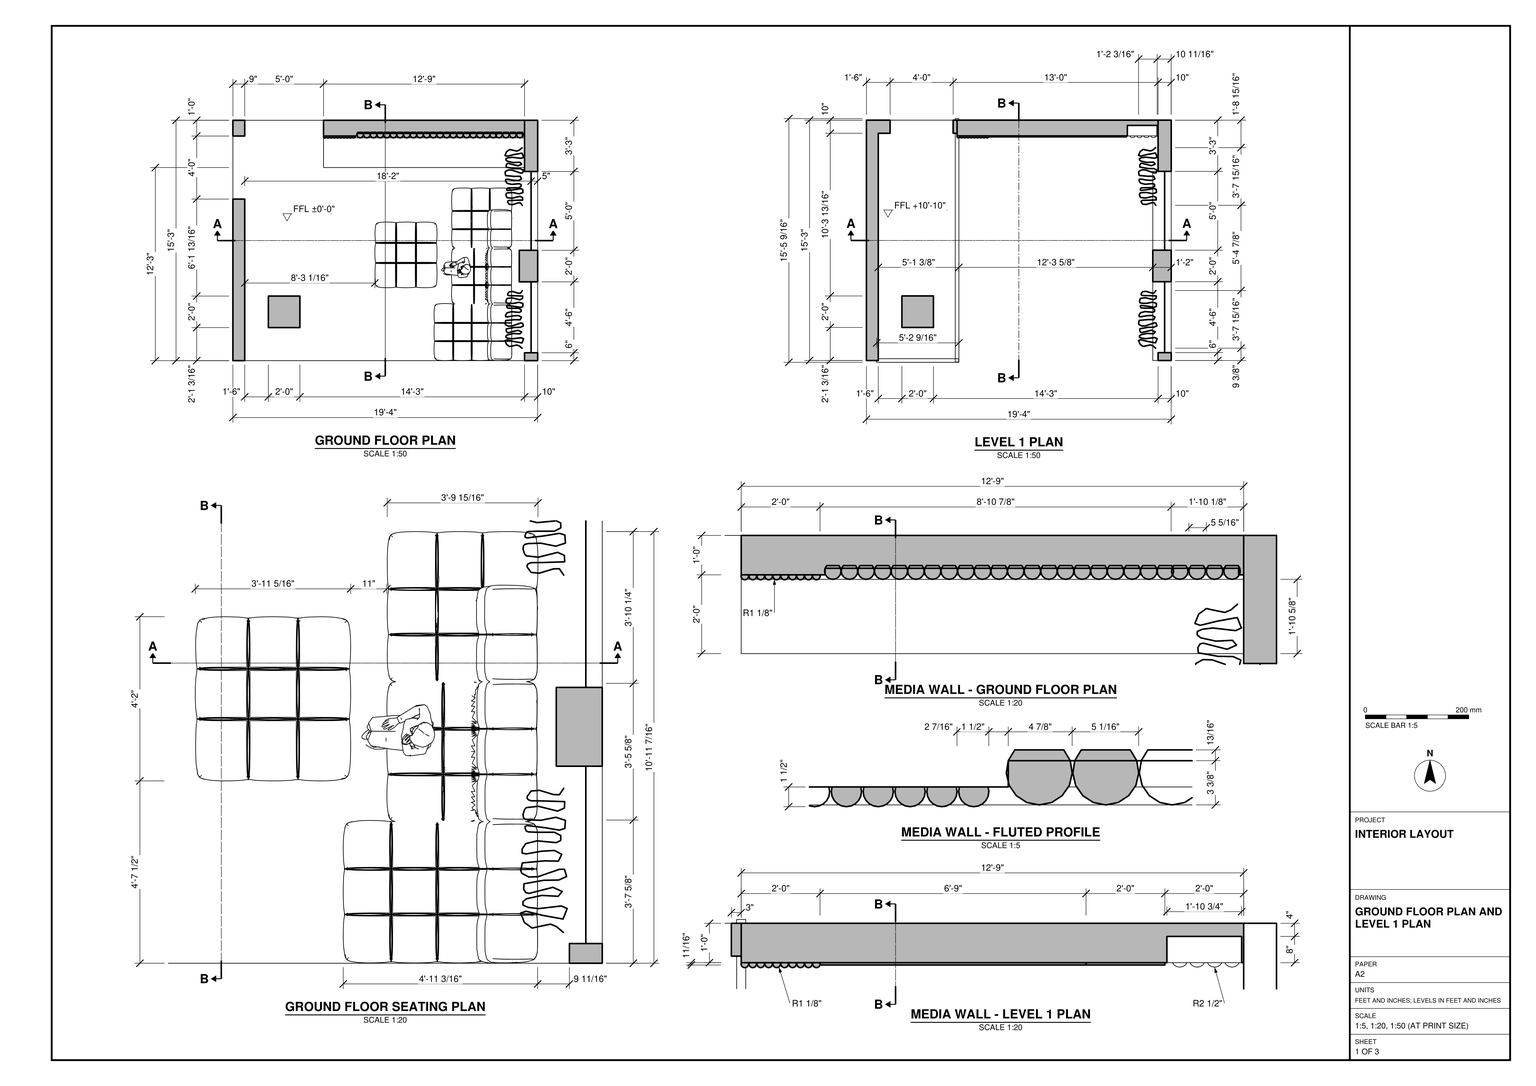
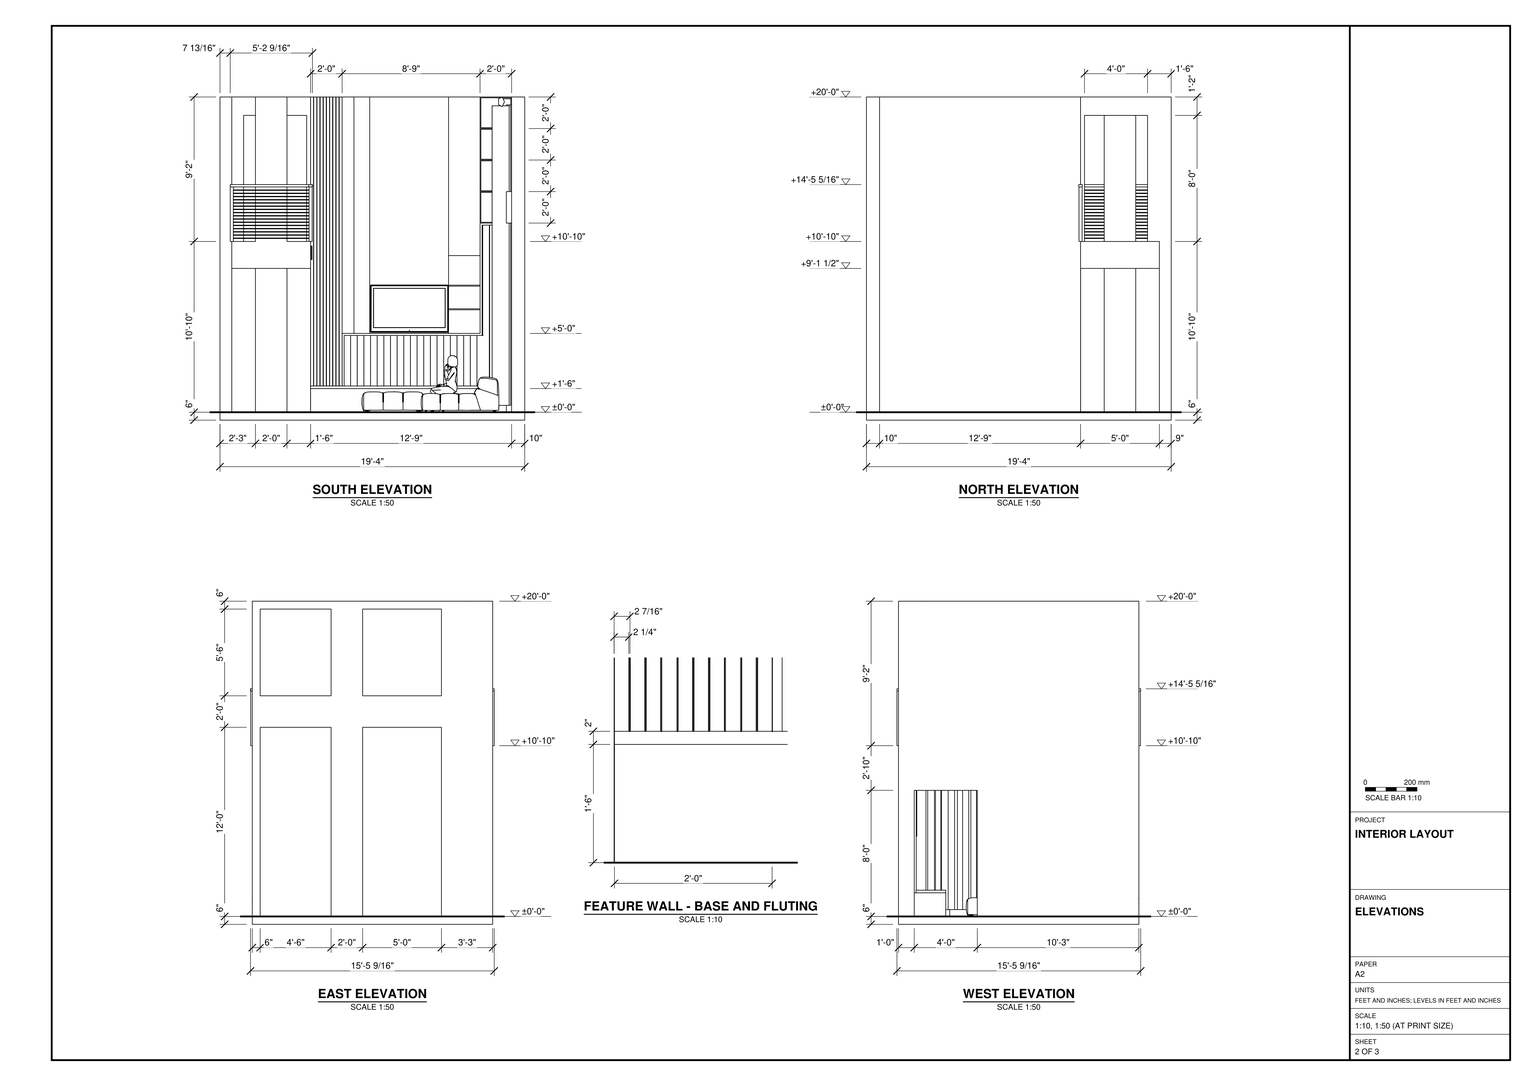
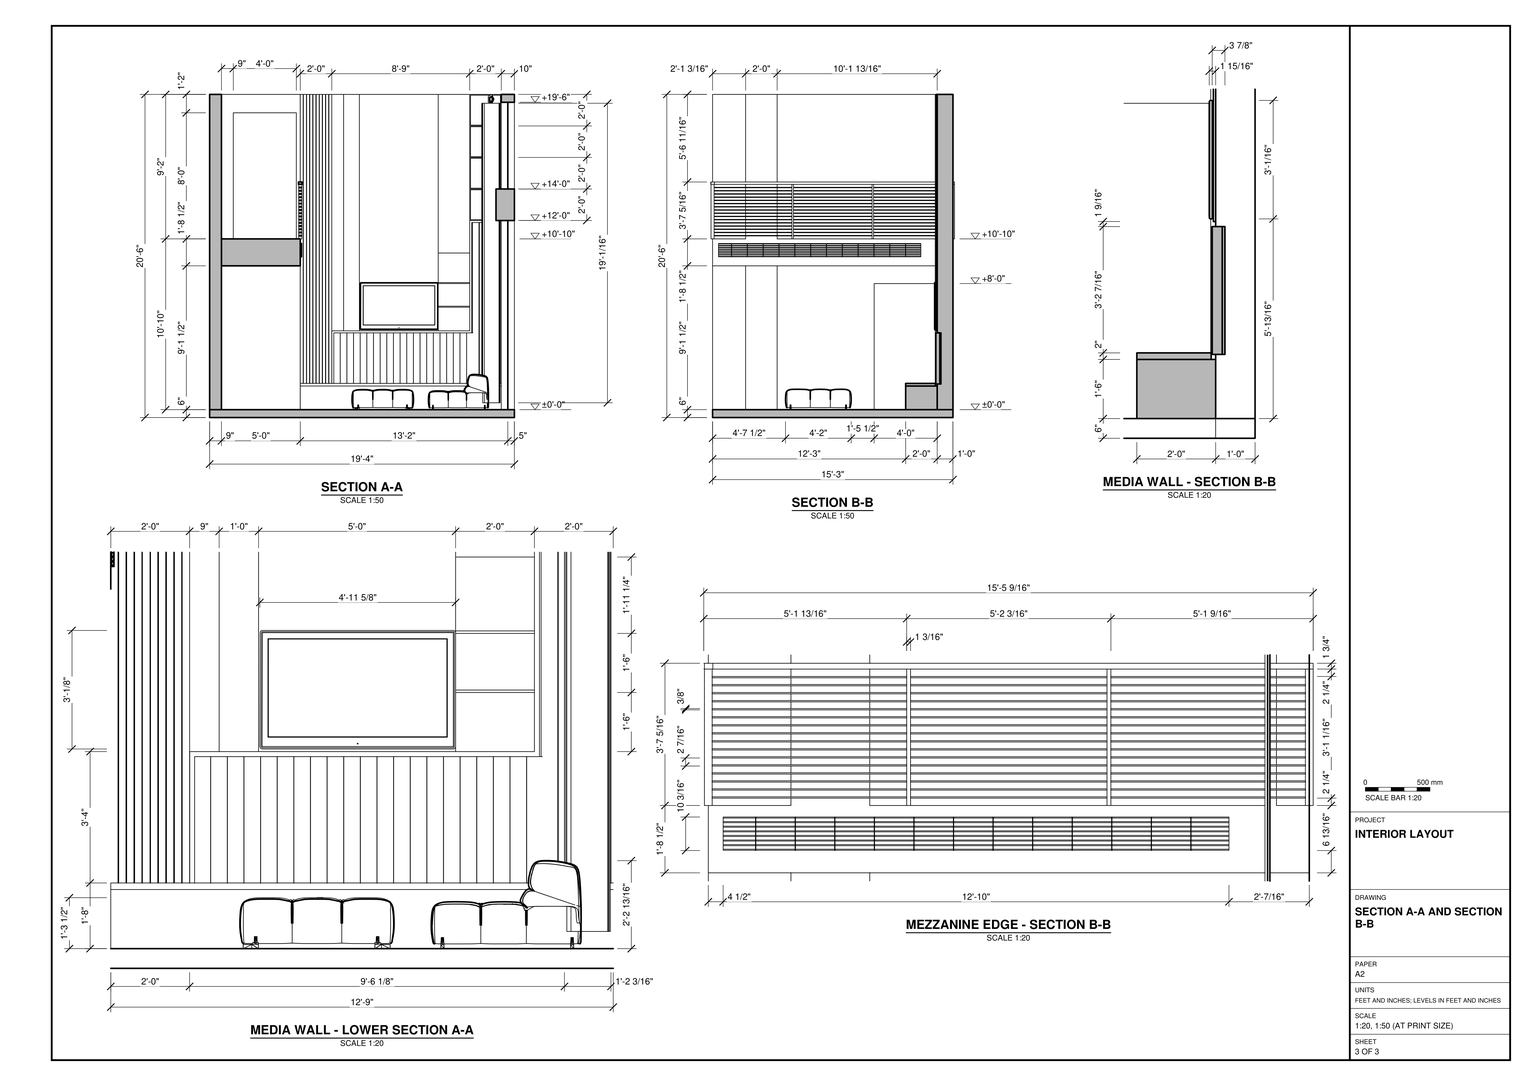
Build the lounge in SketchUp from task_files/diagram_01.pdf. Work in feet and inches. The overall model is 19'-4" wide, 15'-5 9/16" deep and 20'-6" high. Set the ground finished floor at ±0'-0" and the mezzanine finished floor at +10'-10". The overall height includes the 6" ground slab below the finished floor.

Use the plans to locate the walls, their returns and the square column. Match the wall thicknesses and opening sizes to the plans and elevations. Form the narrow mezzanine along the west side, leaving the seating area open to the full room height. Use the mezzanine edge detail to model the horizontal guard rails, their posts and the long grille in the fascia below them.

Build the north media wall in relief. Include the projecting plinth, the narrow full-height fluted strip, the broader flutes below the screen, the tall panels and the shelving beside the screen. Place the long sectional sofa along the east side, with its deeper end as drawn. Leave a gap between the sofa and the separate upholstered ottoman. Decor and loose items, including the curtains and screen, may be any suitable library components.

Keep shell elements and individual furniture or joinery pieces in separate groups or components, and use components for repeated parts. Save one SketchUp model as output_files/double_height_lounge_with_a_mezzanine_and_media_wall.skp.

# SketchUp Ruby script. Lengths in inches.
U = 1.inch
M = Sketchup.active_model
def pt(a) = Geom::Point3d.new(a.map { |v| v * U })
def face(e, loops, mat)
  f = e.add_face(loops[0].map { |a| pt(a) })
  loops[1..].each { |l| e.add_face(l.map { |a| pt(a) }).erase! }
  f.material = f.back_material = mat if mat
  f
end
# faces: each face lists its corners as indices into pts; further lists are holes
def faces(e, pts, list, mat = nil) = list.each { |f| face(e, (f[0].is_a?(Array) ? f : [f]).map { |l| l.map { |i| pts[i] } }, mat) }
# xy, xz, yz: faces in a plane at the given z, y or x. An outline is a flat list of corners, or four numbers for a rectangle; further outlines are holes
def ring(l) = l.size == 4 ? [[l[0], l[1]], [l[2], l[1]], [l[2], l[3]], [l[0], l[3]]] : l.each_slice(2).to_a
def flat(e, list, mat, &to3) = list.each { |f| face(e, (f[0].is_a?(Array) ? f : [f]).map { |l| ring(l).map { |u, v| to3.(u, v) } }, mat) }
def xy(e, z, list, mat = nil) = flat(e, list, mat) { |x, y| [x, y, z] }
def xz(e, y, list, mat = nil) = flat(e, list, mat) { |x, z| [x, y, z] }
def yz(e, x, list, mat = nil) = flat(e, list, mat) { |y, z| [x, y, z] }
def lines(e, pts, list) = list.each { |a, b| e.add_line(pt(pts[a]), pt(pts[b])) }
# prism: a flat outline (further loops are holes) pulled along v
def prism(e, loops, v, mat = nil)
  f = face(e, loops, mat); d = Geom::Vector3d.new(v.map { |x| x * U })
  f.pushpull(f.normal.samedirection?(d) ? d.length : -d.length)
end
def box(e, o, s, mat = nil) = prism(e, [[o, [o[0] + s[0], o[1], o[2]], [o[0] + s[0], o[1] + s[1], o[2]], [o[0], o[1] + s[1], o[2]]]], [0, 0, s[2]], mat)
def at(x, y, z, deg = 0) = Geom::Transformation.translation(pt([x, y, z])) * Geom::Transformation.rotation(ORIGIN, Z_AXIS, deg.degrees)
def axes(o, x, y, z) = Geom::Transformation.new([*x, 0, *y, 0, *z, 0, *pt(o).to_a, 1])
def part(name) = M.definitions.add(name)
# library, detail: a bought-in or finely detailed component or shape, given as its bounding box
def library(name, o, s) = part(name).tap { |d| box(d.entities, o, s) }
def detail(e, o, s) = box(e.add_group.entities, o, s)
def put(e, d, t, mat = nil) = e.add_instance(d, t).tap { |i| i.material = mat if mat }
def group(e, t, mat = nil) = e.add_group.tap { |g| g.transformation = t; g.material = mat if mat }.entities
root = M.entities
M.materials.add("1111 AP 9939 Brown seed-N").color = [122, 81, 68]
M.materials.add("FABRIC ARCHITEX BELLA OLD GOLD").color = [163, 137, 58]
M.materials.add("[Carrera Marble]").color = [206, 206, 206]
M.materials.add("[Color M06]").color = [86, 86, 86]
M.materials.add("[Color M08]").color = [30, 30, 30]
M.materials.add("[Color_D17]").color = [102, 81, 20]
M.materials.add("[Translucent Glass Gray]").color = [128, 128, 128]
M.materials["[Translucent Glass Gray]"].alpha = 0.5
M.materials.add("[Wood Cherry Original]").color = [152, 86, 42]
M.materials.add("[sketch-stone]").color = [126, 99, 107]
c1 = library("Sem nome",[3.92,4.36,0],[38.43,1.9,23.875])
c2 = part("d1")
xy(c2.entities,0,[[0,0,18,1.6],[18,0,36,1.6]],"[sketch-stone]")
xy(c2.entities,72,[[0,0,18,1.6],[18,0,36,1.6]],"[sketch-stone]")
yz(c2.entities,0,[[0,0,1.6,72]],"[sketch-stone]")
yz(c2.entities,36,[[0,0,1.6,72]],"[sketch-stone]")
c3 = part("元件\#28")
box(c3.entities,[0,0.12,0],[0.79,61.77,0.12])
c4 = part("元件\#29")
box(c4.entities,[0,0,0],[0.79,0.2,3.9375])
c5 = part("建立群組\#147")
box(c5.entities,[-0.38,0,0],[0.58,61.77,3.46],"[Color M06]")
c6 = part("建立群組\#1")
put(c6.entities,c3,axes([0,-0.29,0.66],[1.22759,0,0],[0,2.44422,0],[0,0,1.22686]))
put(c6.entities,c3,axes([0,-0.29,0.04],[1.22759,0,0],[0,2.44422,0],[0,0,1.22686]))
put(c6.entities,c4,axes([0.2,139.5625,0],[1.16,0,0],[0,0.66284,0],[0,0,1.16]))
put(c6.entities,c3,axes([0,-0.29,3.8],[1.22759,0,0],[0,2.44422,0],[0,0,1.22686]))
put(c6.entities,c3,axes([0,-0.29,2.55],[1.22759,0,0],[0,2.44422,0],[0,0,1.22686]))
put(c6.entities,c3,axes([0,-0.29,3.18],[1.22759,0,0],[0,2.44422,0],[0,0,1.22686]))
put(c6.entities,c3,axes([0,-0.29,1.29],[1.22759,0,0],[0,2.44422,0],[0,0,1.22686]))
put(c6.entities,c3,axes([0,-0.29,4.43],[1.22759,0,0],[0,2.44422,0],[0,0,1.22686]))
put(c6.entities,c3,axes([0,-0.29,1.92],[1.22759,0,0],[0,2.44422,0],[0,0,1.22686]))
put(c6.entities,c4,axes([0.2,80.51,0],[1.16,0,0],[0,0.66284,0],[0,0,1.16]))
put(c6.entities,c4,axes([0.2,56.88,0],[1.16,0,0],[0,0.66284,0],[0,0,1.16]))
put(c6.entities,c4,axes([0.2,45.07,0],[1.16,0,0],[0,0.66284,0],[0,0,1.16]))
put(c6.entities,c4,axes([0.2,21.45,0],[1.16,0,0],[0,0.66284,0],[0,0,1.16]))
put(c6.entities,c4,axes([0.2,127.75,0],[1.16,0,0],[0,0.66284,0],[0,0,1.16]))
put(c6.entities,c4,axes([0.2,115.9375,0],[1.16,0,0],[0,0.66284,0],[0,0,1.16]))
put(c6.entities,c4,axes([0.2,68.7,0],[1.16,0,0],[0,0.66284,0],[0,0,1.16]))
put(c6.entities,c4,axes([0.2,33.26,0],[1.16,0,0],[0,0.66284,0],[0,0,1.16]))
put(c6.entities,c4,axes([0.2,9.64,0],[1.16,0,0],[0,0.66284,0],[0,0,1.16]))
put(c6.entities,c4,axes([0.2,92.32,0],[1.16,0,0],[0,0.66284,0],[0,0,1.16]))
put(c6.entities,c4,axes([0.2,104.13,0],[1.16,0,0],[0,0.66284,0],[0,0,1.16]))
put(c6.entities,c5,axes([0.72,0,0.18],[1.22759,0,0],[0,2.44422,0],[0,0,1.22686]))
c7 = part("元件\#23")
put(c7.entities,c6,at(-0.03,-11.6875,0))
c8 = library("skpcyxm1p",[14.43,-75.28,0],[105.19,111.11,34.48])
c9 = part("Group\#13")
p = [[0,1.89,0.38],[0,1.89,1.61],[0,0.72,0],[0,0,0.99],[0,0.72,1.99]]
lines(c9.entities,p,[[0,1],[2,0],[3,2],[4,3],[1,4]])
c10 = part("Pleated curtain panel")
xz(c10.entities,0.39,[[4.6,0,5.13,80]],"FABRIC ARCHITEX BELLA OLD GOLD")
xz(c10.entities,1.09,[[22.32,0,22.65,80]],"FABRIC ARCHITEX BELLA OLD GOLD")
xz(c10.entities,6.2,[[20.18,0,20.22,80]],"FABRIC ARCHITEX BELLA OLD GOLD")
yz(c10.entities,16.67,[[2.72,0,5.62,80]],"FABRIC ARCHITEX BELLA OLD GOLD")
yz(c10.entities,22.93,[[5.5,0,6.45,80]],"FABRIC ARCHITEX BELLA OLD GOLD")
p = [[1.66,0.63,0],[3.22,0,0],[3.22,0,80],[1.66,0.63,80],[3.53,0.9,0],[3.53,0.9,80],
  [9.86,0.18,0],[10.31,0.02,0],[10.31,0.02,80],[9.86,0.18,80],[11.57,0.28,0],[11.57,0.28,80],
  [9.23,1.35,0],[9.23,1.35,80],[13.2,0.26,0],[13.86,0.23,0],[13.86,0.23,80],[13.2,0.26,80],
  [14.78,0.86,0],[14.78,0.86,80],[11.91,3.96,0],[11.91,3.96,80],[13.07,0.91,0],[13.07,0.91,80],
  [4.47,0.55,0],[4.6,0.39,0],[4.6,0.39,80],[4.47,0.55,80],[5.13,0.39,0],[5.61,0.97,0],
  [5.61,0.97,80],[5.13,0.39,80],[19.11,0.47,0],[19.64,0.4,0],[19.64,0.4,80],[19.11,0.47,80],
  [20.45,0.65,0],[20.45,0.65,80],[4.17,1.27,0],[4.17,1.27,80],[6.63,0.86,0],[7.21,0.5,0],
  [7.21,0.5,80],[6.63,0.86,80],[8.1,0.56,0],[8.1,0.56,80],[18.86,0.71,0],[18.86,0.71,80],
  [0.73,1.92,0],[0.73,1.92,80],[8.6875,3.87,0],[8.6875,3.87,80],[17.27,0.77,0],[17.64,0.73,0],
  [17.64,0.73,80],[17.27,0.77,80],[17.8,1.0625,0],[17.8,1.0625,80],[18.73,1.28,0],[18.73,1.28,80],
  [20.78,0.94,0],[20.78,0.94,80],[16.86,0.97,0],[16.86,0.97,80],[2.85,3.66,0],[2.85,3.66,80],
  [6.49,1.39,0],[6.49,1.39,80],[13.52,3.45,0],[13.52,3.45,80],[15.24,2.74,0],[15.24,2.74,80],
  [21,2.94,0],[21,2.94,80],[6.16,3.51,0],[6.16,3.51,80],[16.73,1.29,0],[16.73,1.29,80],
  [17.43,4.08,0],[17.43,4.08,80],[22.08,1.29,0],[22.32,1.09,0],[22.32,1.09,80],[22.08,1.29,80],
  [22.65,1.09,0],[23.54,1.75,0],[23.54,1.75,80],[22.65,1.09,80],[3.97,2.98,0],[3.97,2.98,80],
  [9.28,2.9,0],[9.28,2.9,80],[16.67,2.72,0],[16.67,2.72,80],[18.67,3.36,0],[18.67,3.36,80],
  [21.91,1.77,0],[21.91,1.77,80],[7.51,5.37,0],[7.51,5.37,80],[21.89,3.53,0],[21.89,3.53,80],
  [23.65,3.14,0],[23.65,3.14,80],[0.95,2.86,0],[0.95,2.86,80],[14.95,5.92,0],[14.95,5.92,80],
  [1.38,4.99,0],[1.38,4.99,80],[10.52,6.48,0],[10.52,6.48,80],[20.18,6.2,0],[20.18,6.2,80],
  [4.41,6.76,0],[4.41,6.76,80],[22.93,5.5,0],[22.93,5.5,80],[13.64,5.62,0],[13.64,5.62,80],
  [19.17,5.86,0],[19.17,5.86,80],[6.02,6.25,0],[6.02,6.25,80],[21.77,7.33,0],[21.77,7.33,80],
  [2.23,7.06,0],[2.23,7.06,80],[8.72,6.33,0],[8.72,6.33,80],[11.87,6.29,0],[11.87,6.29,80],
  [17.03,6.45,0],[17.03,6.45,80],[0.95,6.01,0],[0.95,6.01,80],[6.82,6.92,0],[6.82,6.92,80],
  [13.01,6.84,0],[13.01,6.84,80],[16.125,6.68,0],[16.67,5.62,0],[16.67,5.62,80],[16.125,6.68,80],
  [15.31,6.67,0],[15.31,6.67,80],[18.65,7.45,0],[18.65,7.45,80],[0,7.11,0],[0,7.11,80],
  [20.22,6.2,0],[20.71,7.28,0],[20.71,7.28,80],[20.22,6.2,80],[9.31,7.65,0],[9.31,7.65,80],
  [17.3,7.35,80],[17.3,7.35,0],[22.93,6.45,0],[24,7.18,0],[24,7.18,80],[22.93,6.45,80],
  [10.5,7.3,0],[10.5,7.3,80],[3.98,7.74,0],[3.98,7.74,80]]
faces(c10.entities,p,[[0,1,2,3],[1,4,5,2],[6,7,8,9],[7,10,11,8],[12,6,9,13],[14,15,16,17],[15,18,19,16],[10,20,21,11],
  [22,14,17,23],[24,25,26,27],[28,29,30,31],[32,33,34,35],[33,36,37,34],[38,24,27,39],[40,41,42,43],[41,44,45,42],
  [46,32,35,47],[48,0,3,49],[44,50,51,45],[52,53,54,55],[53,56,57,54],[58,46,47,59],[36,60,61,37],[62,52,55,63],
  [4,64,65,5],[66,40,43,67],[68,22,23,69],[18,70,71,19],[60,72,73,61],[29,74,75,30],[76,62,63,77],[56,78,79,57],
  [80,81,82,83],[84,85,86,87],[88,38,39,89],[90,12,13,91],[92,76,77,93],[94,58,59,95],[96,80,83,97],[98,66,67,99],
  [100,96,97,101],[85,102,103,86],[104,48,49,105],[70,106,107,71],[108,104,105,109],[110,90,91,111],[72,112,113,73],[114,88,89,115],
  [102,116,117,103],[118,68,69,119],[120,94,95,121],[74,122,123,75],[124,100,101,125],[64,126,127,65],[50,128,129,51],[20,130,131,21],
  [78,132,133,79],[134,108,109,135],[136,98,99,137],[138,118,119,139],[140,141,142,143],[106,144,145,107],[146,120,121,147],[148,134,135,149],
  [122,136,137,123],[150,151,152,153],[128,154,155,129],[130,138,139,131],[156,133,132,157],[158,159,160,161],[162,110,111,163],[144,140,143,145],
  [164,114,115,165],[126,164,165,127],[154,162,163,155],[151,124,125,152],[157,146,147,156]],"FABRIC ARCHITEX BELLA OLD GOLD")
put(c10.entities,c9,at(9.77,5.02,80,-180))
put(c10.entities,c9,at(11.91,5.02,80,-180))
put(c10.entities,c9,at(13.54,5.02,80,-180))
put(c10.entities,c9,at(7.29,5.02,80,-180))
put(c10.entities,c9,at(6.18,5.02,80,-180))
put(c10.entities,c9,at(8.69,5.02,80,-180))
put(c10.entities,c9,at(17.42,5.04,80,-180))
put(c10.entities,c9,at(18.86,5.04,80,-180))
put(c10.entities,c9,at(20.65,5.04,80,-180))
put(c10.entities,c9,at(21.87,5.04,80,-180))
put(c10.entities,c9,at(23.29,5.04,80,-180))
put(c10.entities,c9,at(15.09,5.02,80,-180))
put(c10.entities,c9,at(16.66,5.04,80,-180))
put(c10.entities,c9,at(2.54,5.02,80,-180))
put(c10.entities,c9,at(1.38,5.02,80,-180))
put(c10.entities,c9,at(4.1,5.02,80,-180))
c11 = part("end")
yz(c11.entities,0,[[1.28,1.02,0.97,1.12,0.97,1.45,1.28,1.55,1.48,1.28]])
p = [[2,0,0.49],[0,0.97,1.12],[0,1.28,1.02],[2,1.51,0],[4,0.54,0.84],[4,1.38,0.57],
  [0,1.48,1.28],[2,2.44,1.28],[4,1.9,1.28],[2,0,2.08],[0,0.97,1.45],[4,0.54,1.72],
  [0,1.28,1.55],[2,1.51,2.57],[4,1.38,2]]
faces(c11.entities,p,[[0,1,2,3],[4,0,3,5],[3,2,6,7],[3,7,8,5],[0,9,10,1],[4,11,9,0],[6,12,13,7],[7,13,14,8],
  [13,12,10,9],[14,13,9,11]])
c12 = part("Window curtains 2")
xy(c12.entities,4.87,[[4,-1.25,88,-0.36]],"[Color_D17]")
p = [[88,-0.81,3.51],[88,-1.52,4.03],[4,-1.52,4.03],[4,-0.81,3.51],[88,-0.09,4.03],[4,-0.09,4.03],
  [88,-1.25,4.87],[4,-1.25,4.87],[88,-0.36,4.87],[4,-0.36,4.87],[88,0,0],[88,0,3.75]]
faces(c12.entities,p,[[0,1,2,3],[4,0,3,5],[1,6,7,2],[8,4,5,9]],"[Color_D17]")
lines(c12.entities,p,[[10,11]])
put(c12.entities,c10,axes([3.43,-81.89,8.12],[1,0,0],[0,0,-1],[0,1,0]),"FABRIC ARCHITEX BELLA OLD GOLD")
put(c12.entities,c10,axes([86.875,-81.89,8.12],[-1,0,0],[0,0,-1],[0,1,0]),"FABRIC ARCHITEX BELLA OLD GOLD")
put(c12.entities,c11,axes([0,-2.09,5.41],[1,0,0],[0,0,-1],[0,1,0]),"[Color_D17]")
put(c12.entities,c11,axes([92,-2.09,5.41],[-1,0,0],[0,0,-1],[0,1,0]),"[Color_D17]")
c13 = library("sentado 3",[-36.77,87.53,-0.09],[29.95,23.15,54.89])
c14 = part("Railing post")
prism(c14.entities,[[[0.64,4.1875,-38.93],[4.375,4.1875,-38.93],[4.87,3.37,-38.93],[5.02,2.42,-38.93],[4.8,1.49,-38.93],[4.25,0.7,-38.93],[3.45,0.18,-38.93],[2.51,0,-38.93],[1.57,0.18,-38.93],[0.77,0.7,-38.93],[0.22,1.49,-38.93],[0,2.42,-38.93],[0.15,3.37,-38.93]]],[0,0,38.93])
c15 = part("Vertical post")
prism(c15.entities,[[[0.64,4.1875,-122.93],[4.375,4.1875,-122.93],[4.87,3.37,-122.93],[5.02,2.42,-122.93],[4.8,1.49,-122.93],[4.25,0.7,-122.93],[3.45,0.18,-122.93],[2.51,0,-122.93],[1.57,0.18,-122.93],[0.77,0.7,-122.93],[0.22,1.49,-122.93],[0,2.42,-122.93],[0.15,3.37,-122.93]]],[0,0,122.93])
c16 = part("Vertical slat")
prism(c16.entities,[[[0.06,1.5,-240],[2.24,1.5,-240],[2.3,1.15,-240],[2.24,0.79,-240],[2.08,0.47,-240],[1.82,0.22,-240],[1.5,0.06,-240],[1.15,0,-240],[0.79,0.06,-240],[0.47,0.22,-240],[0.22,0.47,-240],[0.06,0.79,-240],[0,1.15,-240]]],[0,0,240])
c17 = part("Group17\#1")
box(c17.entities,[44.33,366.81,136],[2.36,2.36,41.54])
c18 = part("Group18\#1")
box(c18.entities,[44.33,183.81,136],[2.36,2.36,41.54])
c19 = part("Group19\#1")
box(c19.entities,[44.33,306.4,136],[2.36,1.18,41.54])
box(c19.entities,[44.33,245.4,136],[2.36,1.18,41.54])
c20 = part("Group20\#1")
box(c20.entities,[44.14,183.81,177.54],[2.75,185.36,1.77])
c21 = part("Group21\#1")
box(c21.entities,[44.73,184.99,138.25],[1.57,183,0.39])
box(c21.entities,[44.73,184.99,140.69],[1.57,183,0.39])
box(c21.entities,[44.73,184.99,143.13],[1.57,183,0.4])
box(c21.entities,[44.73,184.99,145.58],[1.57,183,0.39])
box(c21.entities,[44.73,184.99,148.02],[1.57,183,0.39])
box(c21.entities,[44.73,184.99,150.46],[1.57,183,0.4])
box(c21.entities,[44.73,184.99,152.91],[1.57,183,0.39])
box(c21.entities,[44.73,184.99,155.35],[1.57,183,0.4])
box(c21.entities,[44.73,184.99,157.8],[1.57,183,0.39])
box(c21.entities,[44.73,184.99,160.24],[1.57,183,0.39])
box(c21.entities,[44.73,184.99,162.68],[1.57,183,0.4])
box(c21.entities,[44.73,184.99,165.125],[1.57,183,0.4])
box(c21.entities,[44.73,184.99,167.57],[1.57,183,0.39])
box(c21.entities,[44.73,184.99,170.01],[1.57,183,0.4])
box(c21.entities,[44.73,184.99,172.46],[1.57,183,0.39])
box(c21.entities,[44.73,184.99,174.9],[1.57,183,0.39])
c22 = part("Group23\#2")
box(c22.entities,[-15.67,183.81,136],[2.36,2.36,41.54])
c23 = part("Group25\#1")
box(c23.entities,[-15.67,183.61,177.54],[62.36,2.76,1.77])
c24 = part("Group25\#2")
box(c24.entities,[-14.49,184.2,138.25],[60,1.58,0.39])
box(c24.entities,[-14.49,184.2,140.69],[60,1.58,0.39])
box(c24.entities,[-14.49,184.2,143.13],[60,1.58,0.4])
box(c24.entities,[-14.49,184.2,145.58],[60,1.58,0.39])
box(c24.entities,[-14.49,184.2,148.02],[60,1.58,0.39])
box(c24.entities,[-14.49,184.2,150.46],[60,1.58,0.4])
box(c24.entities,[-14.49,184.2,152.91],[60,1.58,0.39])
box(c24.entities,[-14.49,184.2,155.35],[60,1.58,0.4])
box(c24.entities,[-14.49,184.2,157.8],[60,1.58,0.39])
box(c24.entities,[-14.49,184.2,160.24],[60,1.58,0.39])
box(c24.entities,[-14.49,184.2,162.68],[60,1.58,0.4])
box(c24.entities,[-14.49,184.2,165.125],[60,1.58,0.4])
box(c24.entities,[-14.49,184.2,167.57],[60,1.58,0.39])
box(c24.entities,[-14.49,184.2,170.01],[60,1.58,0.4])
box(c24.entities,[-14.49,184.2,172.46],[60,1.58,0.39])
box(c24.entities,[-14.49,184.2,174.9],[60,1.58,0.39])
c25 = library("skpD0I6a8",[14.43,-68.68,0],[105.42,143.14,64.75])
c26 = library("skp0QfVtK",[14.45,-36.06,-0.05],[111.77,111,64.8])
c27 = library("Modular sofa section",[0,0,0],[105.41,111.76,64.75])
yz(root,227,[[7.38,6,61.38,150],[85.38,6,145.38,150],[7.38,174,61.38,240],[85.38,174,145.38,240]],"[Translucent Glass Gray]")
p = [[222,145.38,174],[222,145.38,150],[227,67.38,240],[227,67.38,174],[227,67.38,150],[227,67.38,6],
  [227,61.38,6]]
lines(root,p,[[0,1],[2,3],[4,5],[5,6]])
put(root,c1,axes([108.32,164.15,66.79],[1.55092,0,0],[0,1.44,0],[0,0,1.512]))
put(root,c2,axes([4.74,124.38,0],[0,1.33333,0],[-1,0,0],[0,0,1.41667]))
put(root,c7,axes([68.98,17.82,122.29],[1.0201,0,0],[0,1.0201,0],[0,0,2.23188]))
put(root,c2,axes([18,178.38,130],[1.33333,0,0],[0,1,0],[0,0,1.41667]))
put(root,c8,axes([101.57,90.78,6],[0.45,0,0],[0,0.45,0],[0,0,0.45]))
put(root,c12,axes([222,169.74,244.64],[0,-1.83,0],[0,0,2.85041],[-1.83,0,0]))
put(root,c13,axes([188.21,-7.72,5.31],[0.8,0,0],[0,0.8,0],[0,0,0.8]))
g1 = group(root,at(93,1.38,0),"[Carrera Marble]")
box(g1,[-93,0,0],[232,183,6])
g2 = group(root,at(69,172.38,6),"1111 AP 9939 Brown seed-N")
xy(g2,0,[[0,0,153,12]])
xy(g2,19.53,[[25.53,0,151.47,2]])
xy(g2,58.47,[[25.53,0,33,2],[33,0,105,2],[105,0,130.53,2]])
xy(g2,60,[[105,0,129,8]])
xy(g2,78,[[105,0,129,8]])
xy(g2,78.75,[[105,0,129,8]])
xy(g2,96,[[105,0,129,8]])
xy(g2,96.75,[[105,0,129,8]])
xy(g2,119.25,[[105,0,129,8]])
xy(g2,142.47,[[130.53,0,151.47,2]])
xy(g2,144.62,[[129.62,0,152.38,8]],"[Carrera Marble]")
xy(g2,167.38,[[129.62,0,152.38,8]])
xy(g2,168.62,[[129.62,0,152.38,8]],"[Carrera Marble]")
xy(g2,191.38,[[129.62,0,152.38,8]])
xy(g2,192.62,[[129.62,0,152.38,8]],"[Carrera Marble]")
xy(g2,215.38,[[129.62,0,152.38,8]])
xy(g2,216.62,[[129.62,0,152.38,8]],"[Carrera Marble]")
xy(g2,239.38,[[129.62,0,152.38,8]])
xy(g2,240,[[0,0,153,12]])
xz(g2,0,[[0,0,24,240],[24,0,153,18],[[24,18,153,18,153,144,129,144,129,60,24,60],[25.53,19.53,25.53,58.47,130.53,58.47,130.53,142.47,151.47,142.47,151.47,19.53]],[24,60,33,240],[33,60,105,240],
  [105,78,129,78.75],[105,96,129,96.75],[105,119.25,129,240],[[129,144,153,168],[129.62,144.62,152.38,167.38]],[[129,168,153,192],[129.62,168.62,152.38,191.38]],
  [[129,192,153,216],[129.62,192.62,152.38,215.38]],[[129,216,153,240],[129.62,216.62,152.38,239.38]]])
xz(g2,2,[[25.53,19.53,151.47,19.53,151.47,142.47,130.53,142.47,130.53,58.47,25.53,58.47]])
xz(g2,8,[[105,60,129,78.75],[105,78.75,129,96.75],[105,96.75,129,119.25]])
xz(g2,8,[[129.62,144.62,152.38,167.38],[129.62,168.62,152.38,191.38],[129.62,192.62,152.38,215.38],[129.62,216.62,152.38,239.38]],"[Carrera Marble]")
xz(g2,12,[[0,0,153,240]])
yz(g2,0,[[0,0,12,240]])
yz(g2,25.53,[[0,19.53,2,58.47]])
yz(g2,105,[[0,60,8,78.75],[0,78.75,8,96.75],[0,96.75,8,119.25]])
yz(g2,129,[[0,60,8,78.75],[0,78.75,8,96.75],[0,96.75,8,119.25]])
yz(g2,129.62,[[0,144.62,8,167.38],[0,168.62,8,191.38],[0,192.62,8,215.38],[0,216.62,8,239.38]])
yz(g2,130.53,[[0,58.47,2,78],[0,78,2,78.75],[0,78.75,2,96],[0,96,2,96.75],[0,96.75,2,119.25],
  [0,119.25,2,142.47]])
yz(g2,151.47,[[0,19.53,2,142.47]])
yz(g2,152.38,[[0,144.62,8,167.38],[0,168.62,8,191.38],[0,192.62,8,215.38],[0,216.62,8,239.38]])
yz(g2,153,[[0,0,12,240]])
g3 = group(root,at(93,154.38,6),"[Wood Cherry Original]")
box(g3,[-24,-6,0],[153,24,18])
g4 = group(root,at(94.38,171.01,25.53),"1111 AP 9939 Brown seed-N")
put(g4,c14,at(101.27,0,38.93))
put(g4,c14,at(25.32,0,38.93))
put(g4,c14,at(70.89,0,38.93))
put(g4,c14,at(55.7,0,38.93))
put(g4,c14,at(91.14,0,38.93))
put(g4,c15,at(110.95,0,122.93))
put(g4,c15,at(121.56,0,122.93))
put(g4,c15,at(116.25,0,122.93))
put(g4,c15,at(105.64,0,122.93))
put(g4,c14,at(45.57,0,38.93))
put(g4,c14,at(40.51,0,38.93))
put(g4,c14,at(0,0,38.93))
put(g4,c14,at(15.19,0,38.93))
put(g4,c14,at(10.125,0,38.93))
put(g4,c14,at(35.44,0,38.93))
put(g4,c14,at(81.01,0,38.93))
put(g4,c14,at(65.82,0,38.93))
put(g4,c14,at(5.0625,0,38.93))
put(g4,c14,at(60.76,0,38.93))
put(g4,c14,at(75.95,0,38.93))
put(g4,c14,at(86.08,0,38.93))
put(g4,c14,at(50.63,0,38.93))
put(g4,c14,at(20.25,0,38.93))
put(g4,c14,at(96.2,0,38.93))
put(g4,c14,at(30.38,0,38.93))
g5 = group(root,at(93,171.68,66))
xy(g5,0,[[0,0,9,0.7],[9,0,81,0.7]])
xy(g5,59.25,[[81,0,105,0.7]])
xy(g5,180,[[0,0,81,0.7],[81,0,105,0.7]])
xz(g5,0,[[0,0,9,180],[9,0,21,180],[21,0,81,180],[81,59.25,105,180]],"[Carrera Marble]")
xz(g5,0.7,[[0,0,81,180],[81,59.25,105,180]])
yz(g5,0,[[0,0,0.7,180]])
yz(g5,81,[[0,0,0.7,59.25],[0,59.25,0.7,180]])
yz(g5,105,[[0,59.25,0.7,180]])
g6 = group(root,at(68.94,170.88,6),"1111 AP 9939 Brown seed-N")
put(g6,c16,at(0,0,240))
put(g6,c16,at(19.39,0,240))
put(g6,c16,at(2.42,0,240))
put(g6,c16,at(4.85,0,240))
put(g6,c16,at(7.27,0,240))
put(g6,c16,at(12.12,0,240))
put(g6,c16,at(14.54,0,240))
put(g6,c16,at(9.69,0,240))
put(g6,c16,at(16.97,0,240))
put(g6,c16,at(21.8125,0,240))
g7 = group(root,at(93,148.38,24),"[Color M08]")
box(g7,[-24,0,0],[153,22.63,2])
g8 = group(root,at(223,1.38,6))
xy(g8,0,[[-1,0,9,6],[-5,60,-1,84],[-1,60,9,84],[-1,144,9,183]])
xy(g8,144,[[-5,0,-1,6],[-5,6,-1,60],[-1,6,9,60],[-5,84,-1,144],[-1,84,9,144]])
xy(g8,168,[[-5,0,-1,0,-1,6,9,6,9,60,-5,60],[-5,84,9,144]])
xy(g8,234,[[-1,6,9,60],[-5,60,-1,84],[-1,84,9,144]])
xy(g8,240,[[-1,0,9,183]])
xz(g8,0,[[-1,0,9,240],[-5,144,-1,168]])
xz(g8,6,[[-1,0,9,144],[-1,168,9,234]])
xz(g8,60,[[-5,0,9,144],[-5,168,9,234]])
xz(g8,84,[[-5,0,9,144],[-5,168,9,234]])
xz(g8,144,[[-1,0,9,144],[-5,144,-1,168],[-1,168,9,234]])
xz(g8,183,[[-1,0,9,240]])
yz(g8,-5,[[60,0,60,144,0,144,0,168,60,168,60,234,84,234,84,168,144,168,144,144,84,144,84,0]])
yz(g8,-1,[[0,0,6,144],[144,0,144,234,6,234,6,168,0,168,0,240,183,240,183,0]])
yz(g8,9,[[[0,0,6,0,6,144,60,144,60,0,84,0,84,144,144,144,144,0,183,0,183,240,0,240],[84,168,144,234],[6,168,60,234]]])
p = [[-1,84,168],[-1,84,144],[-1,60,168],[-1,60,144]]
lines(g8,p,[[0,1],[2,3]])
g9 = group(root,at(0,1.38,6))
xy(g9,0,[[0,0,9,123],[0,171,9,183]])
xy(g9,96,[[0,123,9,171]])
xy(g9,130,[[9,173,18,183],[66,173,69,183]])
xy(g9,226,[[18,173,66,183]])
xy(g9,240,[[0,0,9,0,9,173,69,173,69,183,0,183]])
xz(g9,0,[[0,0,9,240]])
xz(g9,123,[[0,0,9,96]])
xz(g9,171,[[0,0,9,96]])
xz(g9,173,[[9,130,18,130,18,226,66,226,66,130,69,130,69,240,9,240]])
xz(g9,183,[[0,0,0,240,69,240,69,130,66,130,66,226,18,226,18,130,9,130,9,0]])
yz(g9,0,[[0,0,0,240,183,240,183,0,171,0,171,96,123,96,123,0]])
yz(g9,9,[[0,0,123,0,123,96,171,96,171,0,183,0,183,130,173,130,173,240,0,240]])
yz(g9,18,[[173,130,183,226]])
yz(g9,66,[[173,130,183,226]])
yz(g9,69,[[173,130,183,240]])
g10 = group(root,at(27,26.54,6),"1111 AP 9939 Brown seed-N")
box(g10,[0,0,0],[24,24,240])
g11 = group(root,at(9,1.38,126))
box(g11,[0,0,-10.5],[60,183,20.5])
put(g11,c17,at(14.49,-184.99,-126))
put(g11,c18,at(14.49,-184.99,-126))
put(g11,c19,at(14.49,-184.99,-126))
put(g11,c20,at(14.49,-184.99,-126))
put(g11,c21,at(14.49,-184.99,-126))
put(g11,c22,at(14.49,-184.99,-126))
put(g11,c23,at(14.49,-184.99,-126))
put(g11,c24,at(14.49,-184.99,-126))
g12 = group(root,at(153.11,132.84,6))
put(g12,c25,axes([28.41,-81.89,0.02],[0,-0.4136,0],[0.4136,0,0],[0,0,0.4136]))
put(g12,c26,axes([28.32,-52.2,0.02],[0,0.4136,0],[0.4136,0,0],[0,0,0.4136]))
put(g12,c27,axes([13.3,-45.2,0.02],[0,-0.4136,0],[0.40946,0,0],[0,0,0.4136]))
